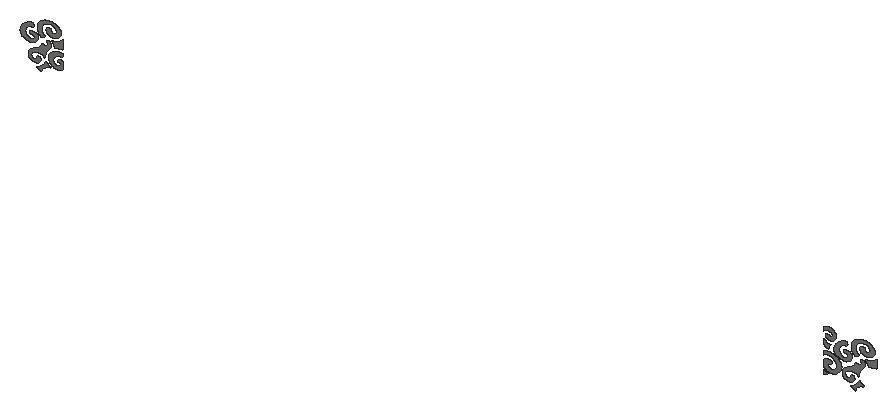
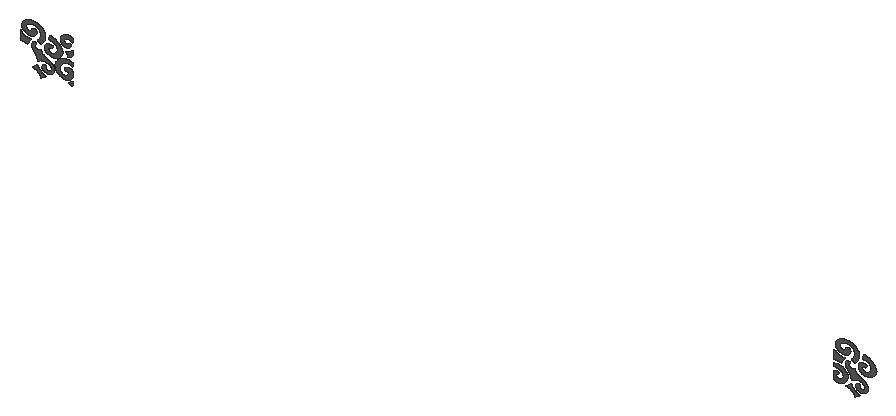
# SketchUp Ruby script. Lengths in inches.
U = 1.inch
M = Sketchup.active_model
def pt(a) = Geom::Point3d.new(a.map { |v| v * U })
def face(e, loops, mat)
  f = e.add_face(loops[0].map { |a| pt(a) })
  loops[1..].each { |l| e.add_face(l.map { |a| pt(a) }).erase! }
  f.material = f.back_material = mat if mat
  f
end
# faces: each face lists its corners as indices into pts; further lists are holes
def faces(e, pts, list, mat = nil) = list.each { |f| face(e, (f[0].is_a?(Array) ? f : [f]).map { |l| l.map { |i| pts[i] } }, mat) }
# xy, xz, yz: faces in a plane at the given z, y or x. An outline is a flat list of corners, or four numbers for a rectangle; further outlines are holes
def ring(l) = l.size == 4 ? [[l[0], l[1]], [l[2], l[1]], [l[2], l[3]], [l[0], l[3]]] : l.each_slice(2).to_a
def flat(e, list, mat, &to3) = list.each { |f| face(e, (f[0].is_a?(Array) ? f : [f]).map { |l| ring(l).map { |u, v| to3.(u, v) } }, mat) }
def xy(e, z, list, mat = nil) = flat(e, list, mat) { |x, y| [x, y, z] }
def xz(e, y, list, mat = nil) = flat(e, list, mat) { |x, z| [x, y, z] }
def yz(e, x, list, mat = nil) = flat(e, list, mat) { |y, z| [x, y, z] }
def lines(e, pts, list) = list.each { |a, b| e.add_line(pt(pts[a]), pt(pts[b])) }
# prism: a flat outline (further loops are holes) pulled along v
def prism(e, loops, v, mat = nil)
  f = face(e, loops, mat); d = Geom::Vector3d.new(v.map { |x| x * U })
  f.pushpull(f.normal.samedirection?(d) ? d.length : -d.length)
end
def box(e, o, s, mat = nil) = prism(e, [[o, [o[0] + s[0], o[1], o[2]], [o[0] + s[0], o[1] + s[1], o[2]], [o[0], o[1] + s[1], o[2]]]], [0, 0, s[2]], mat)
def at(x, y, z, deg = 0) = Geom::Transformation.translation(pt([x, y, z])) * Geom::Transformation.rotation(ORIGIN, Z_AXIS, deg.degrees)
def axes(o, x, y, z) = Geom::Transformation.new([*x, 0, *y, 0, *z, 0, *pt(o).to_a, 1])
def part(name) = M.definitions.add(name)
# library, detail: a bought-in or finely detailed component or shape, given as its bounding box
def library(name, o, s) = part(name).tap { |d| box(d.entities, o, s) }
def detail(e, o, s) = box(e.add_group.entities, o, s)
def put(e, d, t, mat = nil) = e.add_instance(d, t).tap { |i| i.material = mat if mat }
def group(e, t, mat = nil) = e.add_group.tap { |g| g.transformation = t; g.material = mat if mat }.entities
root = M.entities
M.materials.add("[0043_SaddleBrown]4").color = [124, 123, 122]
xz(root,589.17,[[1666.8,173.83,1666.31,174.24,1665.8125,174.64,1665.29,175.02,1664.75,175.39,1664.1875,175.74,1663.61,176.08,1663.01,176.4,1662.4,176.71,1661.77,177,1661.13,177.27,1660.48,177.53,1659.8125,177.77,1661.375,178.34,1662.88,178.99,1664.3125,179.72,1665.67,180.52,1666.95,181.39,1668.14,182.32,1669.23,183.31,1670.22,184.35,1671.11,185.44,1671.89,186.58,1672.55,187.75,1673.1,188.95,1673.65,188.49,1674.21,188.03,1674.78,187.59,1675.36,187.15,1675.95,186.72,1676.55,186.29,1677.17,185.87,1677.79,185.46,1678.41,185.06,1679.05,184.66,1679.7,184.27,1680.36,183.89,1678.69,183.57,1677.08,183.14,1675.54,182.59,1674.08,181.94,1672.71,181.19,1671.46,180.35,1670.32,179.42,1669.32,178.41,1668.46,177.34,1667.74,176.21,1667.19,175.04],[2917.42,173.83,2916.94,174.24,2916.4375,174.64,2915.91,175.02,2915.37,175.39,2914.8125,175.74,2914.23,176.08,2913.64,176.4,2913.03,176.71,2912.4,177,2911.76,177.27,2911.1,177.53,2910.4375,177.77,2912,178.34,2913.5,178.99,2914.9375,179.72,2916.3,180.52,2917.57,181.39,2918.76,182.32,2919.85,183.31,2920.85,184.35,2921.73,185.44,2922.51,186.58,2923.18,187.75,2923.72,188.95,2924.27,188.49,2924.83,188.03,2925.99,187.15,2926.58,186.72,2927.18,186.29,2927.79,185.87,2928.41,185.46,2929.04,185.06,2929.68,184.66,2930.32,184.27,2930.98,183.89,2929.32,183.57,2927.71,183.14,2926.17,182.59,2924.7,181.94,2923.34,181.19,2922.08,180.35,2920.95,179.42,2919.94,178.41,2919.08,177.34,2918.37,176.21,2917.81,175.04],[2869.23,179.89,2869.23,185.26,2869.64,184.92,2870.08,184.6,2870.53,184.3,2871.01,184.01,2871.5,183.73,2872.01,183.47,2872.53,183.23,2873.07,183,2873.62,182.79,2874.18,182.6,2874.76,182.42,2875.34,182.27,2874.96,181.9375,2874.55,181.63,2874.11,181.34,2873.64,181.07,2873.15,180.83,2872.63,180.61,2872.1,180.42,2871.55,180.26,2870.98,180.12,2870.4,180.02,2869.82,179.9375],[1656.02,183.24,1654.59,183.36,1653.2,183.65,1651.89,184.08,1650.68,184.65,1649.61,185.34,1648.69,186.15,1647.96,187.04,1647.42,188.01,1647.09,189.02,1646.98,190.0625,1646.87,191.26,1646.93,192.46,1647.17,193.65,1647.57,194.8125,1648.14,195.9375,1648.86,197.02,1649.74,198.04,1650.76,198.99,1651.91,199.85,1653.18,200.63,1654.56,201.31,1656.02,201.88,1657.41,202.4,1658.74,202.99,1660.02,203.65,1661.22,204.37,1662.35,205.15,1663.4,205.98,1664.37,206.87,1665.25,207.81,1666.03,208.78,1666.71,209.8,1667.3,210.85,1667.77,211.92,1668.45,211.55,1669.19,211.25,1669.98,211.03,1670.81,210.88,1671.65,210.82,1672.5,210.84,1673.34,210.9375,1674.15,211.12,1674.92,211.38,1675.63,211.72,1676.28,212.12,1676.84,212.58,1677.05,212.95,1677.19,213.33,1677.28,213.73,1677.3,214.13,1677.26,214.53,1677.16,214.92,1677,215.3,1676.78,215.67,1676.5,216.02,1676.17,216.34,1675.79,216.63,1675.37,216.89,1675.14,217.04,1674.96,217.23,1674.83,217.43,1674.75,217.65,1674.74,217.875,1674.79,218.1,1674.9,218.3125,1675.07,218.5,1675.28,218.67,1675.53,218.8,1675.82,218.9,1676.12,218.95,1676.68,218.98,1677.23,218.95,1677.78,218.86,1678.3,218.72,1678.79,218.52,1679.23,218.28,1679.625,217.99,1679.96,217.67,1680.22,217.3125,1680.41,216.9375,1680.53,216.54,1680.57,216.14,1680.78,215.47,1680.93,214.79,1681,214.11,1681.01,213.42,1680.95,212.73,1680.82,212.05,1680.62,211.38,1680.35,210.72,1680.02,210.08,1679.62,209.45,1679.16,208.85,1678.64,208.27,1677.71,207.26,1676.84,206.23,1676.03,205.16,1675.29,204.07,1674.63,202.95,1674.03,201.82,1673.51,200.67,1673.05,199.5,1672.68,198.32,1672.375,197.12,1672.15,195.92,1672,194.71,1671.03,195.61,1669.91,196.41,1668.65,197.09,1667.29,197.66,1665.83,198.09,1664.31,198.375,1662.74,198.52,1661.17,198.52,1659.61,198.37,1658.09,198.07,1656.63,197.63,1655.27,197.0625,1654.29,196.53,1653.43,195.9,1652.68,195.2,1652.06,194.44,1651.58,193.625,1651.25,192.77,1651.07,191.9,1651.06,191.01,1651.2,190.14,1651.5,189.28,1651.94,188.46,1652.53,187.68,1653.08,187.38,1653.68,187.15,1654.32,186.98,1654.99,186.89,1655.68,186.87,1656.36,186.92,1657.02,187.04,1657.64,187.24,1658.23,187.5,1658.75,187.82,1659.19,188.1875,1659.5625,188.6,1659.44,188.9,1659.35,189.2,1659.3,189.5,1659.28,189.81,1659.3,190.12,1659.34,190.42,1659.42,190.72,1659.54,191.02,1659.69,191.31,1659.86,191.59,1660.07,191.86,1660.31,192.11,1660.54,192.31,1660.8125,192.48,1661.12,192.61,1661.45,192.71,1661.8,192.77,1662.15,192.79,1662.51,192.77,1662.86,192.71,1663.19,192.61,1663.5,192.48,1663.77,192.31,1664,192.11,1664.67,191.31,1665.15,190.43,1665.4,189.51,1665.4375,188.57,1665.25,187.63,1664.84,186.74,1664.23,185.91,1663.43,185.17,1662.46,184.53,1661.36,184.03,1660.16,183.66,1658.89,183.45,1657.47,183.27],[2906.65,183.24,2905.21,183.36,2903.83,183.65,2902.51,184.08,2901.3,184.65,2900.23,185.34,2899.32,186.15,2898.58,187.04,2898.04,188.01,2897.72,189.02,2897.61,190.0625,2897.49,191.26,2897.56,192.46,2897.79,193.65,2898.19,194.8125,2898.76,195.9375,2899.49,197.02,2900.37,198.04,2901.39,198.99,2902.54,199.85,2903.81,200.63,2905.18,201.31,2906.65,201.88,2908.04,202.4,2909.37,202.99,2910.64,203.65,2911.85,204.37,2912.98,205.15,2914.03,205.98,2914.99,206.87,2915.87,207.81,2916.65,208.78,2917.34,209.8,2917.92,210.85,2918.4,211.92,2919.08,211.55,2919.82,211.25,2920.61,211.03,2921.43,210.88,2922.28,210.82,2923.13,210.84,2923.97,210.9375,2924.78,211.12,2925.55,211.38,2926.26,211.72,2926.9,212.12,2927.47,212.58,2927.67,212.95,2927.82,213.33,2927.9,213.73,2927.93,214.13,2927.89,214.53,2927.78,214.92,2927.62,215.3,2927.4,215.67,2927.125,216.02,2926.79,216.34,2926.42,216.63,2926,216.89,2925.77,217.04,2925.58,217.23,2925.45,217.43,2925.38,217.65,2925.37,217.875,2925.42,218.1,2925.53,218.3125,2925.69,218.5,2925.9,218.67,2926.16,218.8,2926.44,218.9,2926.75,218.95,2927.3,218.98,2927.86,218.95,2928.4,218.86,2928.93,218.72,2929.41,218.52,2929.86,218.28,2930.25,217.99,2930.58,217.67,2930.85,217.3125,2931.04,216.9375,2931.16,216.54,2931.19,216.14,2931.41,215.47,2931.55,214.79,2931.63,214.11,2931.64,213.42,2931.57,212.73,2931.44,212.05,2931.24,211.38,2930.98,210.72,2930.64,210.08,2930.24,209.45,2929.79,208.85,2929.27,208.27,2928.33,207.26,2927.46,206.23,2926.66,205.16,2925.92,204.07,2925.25,202.95,2924.66,201.82,2924.13,200.67,2923.68,199.5,2923.3,198.32,2923,197.12,2922.77,195.92,2922.62,194.71,2921.65,195.61,2920.53,196.41,2919.28,197.09,2917.91,197.66,2916.45,198.09,2914.93,198.375,2913.37,198.52,2911.79,198.52,2910.23,198.37,2908.71,198.07,2907.26,197.63,2905.89,197.0625,2904.92,196.53,2904.05,195.9,2903.3,195.2,2902.68,194.44,2902.2,193.625,2901.875,192.77,2901.7,191.9,2901.68,191.01,2901.82,190.14,2902.12,189.28,2902.57,188.46,2903.16,187.68,2903.7,187.38,2904.31,187.15,2904.95,186.98,2905.62,186.89,2906.3,186.87,2906.98,186.92,2907.64,187.04,2908.27,187.24,2908.85,187.5,2909.37,187.82,2909.82,188.1875,2910.1875,188.6,2910.07,188.9,2909.98,189.2,2909.93,189.5,2909.91,189.81,2909.92,190.12,2909.97,190.42,2910.05,190.72,2910.16,191.02,2910.31,191.31,2910.49,191.59,2910.7,191.86,2910.93,192.11,2911.16,192.31,2911.4375,192.48,2911.74,192.61,2912.07,192.71,2912.42,192.77,2912.78,192.79,2913.14,192.77,2913.48,192.71,2913.82,192.61,2914.12,192.48,2914.39,192.31,2914.625,192.11,2915.3,191.31,2915.77,190.43,2916.03,189.51,2916.0625,188.57,2915.875,187.63,2915.47,186.74,2914.85,185.91,2914.05,185.17,2913.09,184.53,2911.99,184.03,2910.78,183.66,2909.51,183.45,2908.09,183.27],
  [2879.38,184.38,2878.22,184.54,2877.08,184.78,2875.99,185.09,2874.9375,185.48,2873.94,185.94,2873.01,186.47,2872.16,187.05,2871.38,187.69,2870.7,188.38,2870.11,189.12,2869.61,189.89,2869.23,190.7,2869.23,198.78,2869.76,199.6875,2870.53,200.5,2871.52,201.17,2872.68,201.69,2873.96,202.03,2875.3,202.17,2876.67,202.12,2877.98,201.86,2879.2,201.42,2880.26,200.8,2881.13,200.05,2881.77,199.18,2881.87,198.97,2881.92,198.75,2881.92,198.53,2881.88,198.32,2881.8,198.1,2881.67,197.9,2881.51,197.72,2881.31,197.55,2881.07,197.41,2880.82,197.3,2880.54,197.21,2880.24,197.15,2879.51,197.24,2878.78,197.23,2878.06,197.13,2877.375,196.93,2876.75,196.64,2876.22,196.28,2875.78,195.85,2875.47,195.37,2875.28,194.85,2875.22,194.32,2875.31,193.8,2875.52,193.29,2875.7,192.63,2876.03,192,2876.49,191.41,2877.07,190.88,2877.76,190.43,2878.53,190.06,2879.38,189.78,2880.28,189.6,2881.21,189.53,2882.14,189.5625,2883.06,189.7,2883.93,189.9375,2885.28,190.72,2886.47,191.64,2887.47,192.67,2888.25,193.79,2888.8125,194.98,2889.13,196.21,2889.2,197.47,2889.03,198.72,2888.61,199.93,2887.96,201.1,2887.09,202.18,2886.01,203.17,2885.57,203.82,2885.06,204.45,2884.47,205.04,2883.83,205.59,2883.12,206.1,2882.35,206.57,2881.53,206.99,2880.67,207.37,2879.76,207.68,2878.82,207.94,2877.86,208.15,2876.875,208.3,2876.17,208.36,2875.47,208.375,2874.76,208.35,2874.0625,208.28,2873.37,208.17,2872.7,208.02,2872.04,207.83,2871.41,207.6,2870.8125,207.33,2870.24,207.03,2869.71,206.69,2869.23,206.32,2869.23,211.9,2871.37,212.41,2873.59,212.74,2875.84,212.875,2878.1,212.8125,2880.34,212.56,2882.51,212.11,2884.6,211.48,2886.5625,210.67,2888.38,209.7,2890.02,208.58,2891.47,207.33,2892.7,205.96,2894.37,203.92,2895.52,201.7,2896.14,199.375,2896.18,197.01,2895.66,194.67,2894.59,192.43,2893,190.36,2890.9375,188.51,2888.46,186.95,2885.66,185.72,2882.6,184.86],[1691.55,185,1690.19,185.0625,1688.86,185.24,1687.5625,185.54,1686.33,185.94,1685.17,186.46,1684.11,187.07,1683.22,187.69,1682.38,188.36,1681.61,189.0625,1680.91,189.8,1680.28,190.57,1679.72,191.375,1679.23,192.2,1678.83,193.05,1678.5,193.92,1678.26,194.79,1678.09,195.68,1678.01,196.58,1678.13,198.46,1678.64,200.32,1679.53,202.09,1680.78,203.75,1682.36,205.26,1684.24,206.58,1686.37,207.67,1688.7,208.53,1691.19,209.12,1693.78,209.4375,1696.39,209.47,1698.99,209.22,1698.99,204.51,1696.76,204.57,1694.55,204.34,1692.43,203.84,1690.46,203.08,1688.71,202.09,1687.22,200.89,1686.04,199.53,1685.21,198.03,1684.75,196.46,1684.67,194.85,1684.99,193.26,1685.6875,191.73,1686.48,191.08,1687.43,190.54,1688.51,190.15,1689.67,189.91,1690.87,189.83,1692.07,189.91,1693.23,190.16,1694.3,190.55,1695.25,191.09,1696.04,191.75,1696.65,192.5,1697.05,193.32,1697.125,193.65,1697.12,193.99,1697.03,194.32,1696.87,194.64,1696.63,194.93,1696.33,195.19,1695.97,195.4,1695.5625,195.57,1695.125,195.6875,1694.66,195.75,1694.2,195.75,1693.73,195.7,1693.49,195.77,1693.26,195.87,1693.05,195.98,1692.86,196.11,1692.68,196.25,1692.53,196.41,1692.4,196.58,1692.3,196.75,1692.22,196.93,1692.17,197.12,1692.15,197.3125,1692.16,197.5,1692.53,197.89,1692.97,198.24,1693.46,198.54,1694.01,198.8,1694.6,199,1695.23,199.14,1695.87,199.22,1696.52,199.24,1697.17,199.19,1697.8,199.09,1698.42,198.93,1698.99,198.7,1698.99,187.07,1697.93,186.46,1696.77,185.94,1695.54,185.54,1694.24,185.24,1692.91,185.0625],[1649.44,208.61,1647.11,208.71,1644.82,209.07,1642.64,209.68,1640.62,210.53,1638.8125,211.6,1637.25,212.86,1635.99,214.28,1635.04,215.82,1634.44,217.45,1634.2,219.125,1634.33,220.81,1634.82,222.46,1635.375,224.06,1636.13,225.62,1637.08,227.12,1638.22,228.55,1639.54,229.9,1641.02,231.16,1642.66,232.31,1644.44,233.35,1646.34,234.27,1648.35,235.06,1650.45,235.71,1652.625,236.22,1653.04,235.77,1653.4,235.31,1653.71,234.82,1653.98,234.32,1654.1875,233.81,1654.34,233.28,1654.44,232.75,1654.49,232.22,1654.48,231.68,1654.41,231.15,1654.29,230.62,1654.12,230.1,1652.76,230.21,1651.4,230.19,1650.06,230.04,1648.76,229.75,1647.53,229.33,1646.38,228.8,1645.36,228.16,1644.46,227.42,1643.71,226.6,1643.13,225.71,1642.72,224.77,1642.5,223.8,1642.13,222.89,1641.9,221.95,1641.8125,221,1641.87,220.05,1642.06,219.11,1642.39,218.19,1642.86,217.3,1643.45,216.45,1644.17,215.65,1645.01,214.91,1645.94,214.24,1646.98,213.65,1647.93,213.25,1648.98,212.99,1650.07,212.875,1651.18,212.91,1652.25,213.1,1653.26,213.43,1654.16,213.89,1654.93,214.46,1655.53,215.13,1655.94,215.875,1656.16,216.66,1656.16,217.45,1656.07,217.85,1655.91,218.23,1655.68,218.59,1655.38,218.92,1655.03,219.23,1654.61,219.49,1654.16,219.71,1653.66,219.89,1653.14,220.01,1652.6,220.09,1652.04,220.1,1651.49,220.07,1650.92,220.05,1650.36,220.13,1649.83,220.3,1649.37,220.55,1649,220.86,1648.75,221.23,1648.61,221.63,1648.61,222.05,1648.73,222.45,1648.98,222.83,1649.34,223.15,1649.79,223.4,1651.04,223.84,1652.38,224.12,1653.76,224.21,1655.14,224.12,1656.48,223.85,1657.73,223.4,1658.84,222.81,1659.79,222.07,1660.53,221.23,1661.06,220.3,1661.33,219.32,1661.36,218.32,1661.41,217.11,1661.24,215.9,1660.83,214.72,1660.21,213.6,1659.375,212.54,1658.35,211.58,1657.15,210.73,1655.8,210.01,1654.33,209.42,1652.76,208.99,1651.12,208.72],[2900.07,208.61,2897.73,208.71,2895.45,209.07,2893.27,209.68,2891.25,210.53,2889.4375,211.6,2887.88,212.86,2886.61,214.28,2885.67,215.82,2885.07,217.45,2884.83,219.125,2884.96,220.81,2885.45,222.46,2886,224.06,2886.76,225.62,2887.71,227.12,2888.85,228.55,2890.16,229.9,2891.65,231.16,2893.28,232.31,2895.06,233.35,2896.96,234.27,2898.97,235.06,2901.07,235.71,2903.25,236.22,2903.66,235.77,2904.03,235.31,2904.34,234.82,2904.6,234.32,2904.8125,233.81,2904.97,233.28,2905.07,232.75,2905.11,232.22,2905.1,231.68,2905.04,231.15,2904.92,230.62,2904.74,230.1,2903.39,230.21,2902.03,230.19,2900.69,230.04,2899.38,229.75,2898.15,229.33,2897.01,228.8,2895.98,228.16,2895.08,227.42,2894.34,226.6,2893.76,225.71,2893.35,224.77,2893.125,223.8,2892.76,222.89,2892.53,221.95,2892.4375,221,2892.49,220.05,2892.68,219.11,2893.02,218.19,2893.48,217.3,2894.08,216.45,2894.8,215.65,2895.63,214.91,2896.57,214.24,2897.6,213.65,2898.56,213.25,2899.6,212.99,2900.7,212.875,2901.8,212.91,2902.875,213.1,2903.88,213.43,2904.79,213.89,2905.55,214.46,2906.15,215.13,2906.57,215.875,2906.78,216.66,2906.78,217.45,2906.7,217.85,2906.54,218.23,2906.31,218.59,2906.01,218.92,2905.65,219.23,2905.24,219.49,2904.78,219.71,2904.29,219.89,2903.76,220.01,2903.22,220.09,2902.67,220.1,2902.12,220.07,2901.55,220.05,2900.98,220.13,2900.46,220.3,2900,220.55,2899.63,220.86,2899.37,221.23,2899.24,221.63,2899.23,222.05,2899.36,222.45,2899.61,222.83,2899.97,223.15,2900.42,223.4,2901.66,223.84,2903,224.12,2904.39,224.21,2905.77,224.12,2907.11,223.85,2908.35,223.4,2909.47,222.81,2910.41,222.07,2911.16,221.23,2911.68,220.3,2911.96,219.32,2911.98,218.32,2912.04,217.11,2911.86,215.9,2911.46,214.72,2910.83,213.6,2910,212.54,2908.98,211.58,2907.78,210.73,2906.43,210.01,2904.95,209.42,2903.38,208.99,2901.74,208.72],[1687.01,213.07,1686.91,213.85,1686.75,214.62,1686.53,215.39,1686.27,216.14,1685.95,216.89,1685.57,217.625,1685.15,218.34,1684.68,219.05,1684.15,219.73,1683.58,220.4,1682.97,221.04,1682.31,221.66,1683.96,221.55,1685.62,221.5625,1687.27,221.7,1688.89,221.96,1690.47,222.33,1691.99,222.82,1693.43,223.41,1694.78,224.11,1696.02,224.91,1697.14,225.79,1698.14,226.75,1698.99,227.78,1698.99,215.23,1697.95,215.21,1696.92,215.16,1695.88,215.08,1694.85,214.98,1693.83,214.84,1692.82,214.67,1691.82,214.47,1690.83,214.25,1689.85,213.99,1688.89,213.71,1687.9375,213.41],
  [2937.63,213.07,2937.53,213.85,2937.37,214.62,2937.16,215.39,2936.89,216.14,2936.57,216.89,2936.2,217.625,2935.78,218.34,2935.3,219.05,2934.78,219.73,2934.21,220.4,2933.59,221.04,2932.93,221.66,2934.59,221.55,2936.25,221.5625,2937.9,221.7,2939.52,221.96,2941.1,222.33,2942.61,222.82,2944.05,223.41,2945.4,224.11,2946.64,224.91,2947.77,225.79,2948.76,226.75,2949.62,227.78,2949.62,215.23,2948.58,215.21,2947.54,215.16,2946.51,215.08,2945.48,214.98,2944.46,214.84,2943.45,214.67,2942.44,214.47,2941.45,214.25,2940.47,213.99,2939.51,213.71,2938.5625,213.41],[2876.57,216.375,2875.87,216.63,2875.19,216.91,2874.51,217.2,2873.86,217.52,2873.22,217.84,2872.59,218.1875,2871.98,218.54,2871.39,218.92,2870.82,219.31,2870.27,219.71,2869.74,220.125,2869.23,220.56,2869.23,227.67,2869.75,227.04,2870.34,226.43,2870.99,225.86,2871.71,225.34,2872.49,224.85,2873.32,224.42,2874.19,224.03,2875.11,223.7,2876.06,223.42,2877.03,223.2,2878.03,223.04,2879.05,222.93,2878.63,222.44,2878.25,221.9375,2877.9,221.42,2877.6,220.89,2877.33,220.35,2877.1,219.79,2876.91,219.23,2876.76,218.67,2876.65,218.1,2876.58,217.52,2876.55,216.95],[1666.39,220.74,1665.27,221.82,1664.26,222.95,1663.37,224.13,1662.6,225.36,1661.97,226.63,1661.46,227.92,1661.1,229.24,1660.86,230.58,1660.77,231.92,1660.82,233.27,1661,234.61,1661.32,235.94,1661.85,237.37,1662.58,238.75,1663.5,240.07,1664.61,241.32,1665.88,242.48,1667.32,243.55,1668.89,244.5,1670.59,245.33,1672.4,246.03,1674.3,246.59,1676.27,247.02,1678.29,247.29,1680.49,247.4,1682.69,247.29,1684.85,246.97,1686.93,246.4375,1688.89,245.71,1690.7,244.79,1692.31,243.71,1693.71,242.47,1694.86,241.12,1695.74,239.66,1696.34,238.125,1696.64,236.55,1696.64,235.18,1696.36,233.83,1695.8,232.52,1694.99,231.29,1693.93,230.15,1692.66,229.14,1691.19,228.27,1689.57,227.57,1687.82,227.04,1685.98,226.71,1684.09,226.57,1682.2,226.63,1680.72,226.85,1679.32,227.24,1678.02,227.79,1676.87,228.48,1675.89,229.3,1675.11,230.23,1674.54,231.23,1674.22,232.29,1674.14,233.37,1674.3,234.45,1674.71,235.49,1675.35,236.47,1675.87,236.87,1676.48,237.18,1677.17,237.39,1677.91,237.5,1678.66,237.49,1679.4,237.375,1680.09,237.15,1680.69,236.83,1681.2,236.43,1681.57,235.96,1681.81,235.44,1681.7,235.09,1681.64,234.73,1681.63,234.37,1681.6875,234.01,1681.8,233.65,1681.96,233.3125,1682.18,232.98,1682.44,232.68,1682.75,232.39,1683.11,232.13,1683.5,231.91,1683.92,231.71,1684.93,231.82,1685.91,232.03,1686.83,232.35,1687.67,232.77,1688.41,233.28,1689.04,233.86,1689.53,234.5,1689.88,235.19,1690.08,235.91,1690.125,236.65,1690.01,237.38,1689.74,238.09,1689,239.28,1687.99,240.36,1686.74,241.3,1685.29,242.08,1683.6875,242.67,1681.97,243.07,1680.18,243.25,1678.37,243.21,1676.6,242.96,1674.91,242.5,1673.35,241.84,1671.97,241,1670.52,239.82,1669.3,238.51,1668.32,237.1,1667.62,235.6,1667.1875,234.06,1667.04,232.48,1667.1875,230.91,1667.62,229.36,1668.32,227.86,1669.3,226.45,1670.52,225.14,1671.97,223.96,1671.61,223.61,1671.22,223.28,1670.82,222.95,1670.39,222.65,1669.95,222.35,1669.49,222.07,1669.01,221.81,1668.51,221.5625,1668,221.33,1667.48,221.12,1666.94,220.92],[2917.02,220.74,2915.89,221.82,2914.88,222.95,2913.99,224.13,2913.23,225.36,2912.59,226.63,2912.09,227.92,2911.72,229.24,2911.49,230.58,2911.4,231.92,2911.44,233.27,2911.625,234.61,2911.95,235.94,2912.48,237.37,2913.21,238.75,2914.13,240.07,2915.23,241.32,2916.51,242.48,2917.94,243.55,2919.51,244.5,2921.22,245.33,2923.02,246.03,2924.92,246.59,2926.89,247.02,2928.91,247.29,2931.11,247.4,2933.31,247.29,2935.48,246.97,2937.56,246.4375,2939.52,245.71,2941.32,244.79,2942.94,243.71,2944.33,242.47,2945.48,241.12,2946.36,239.66,2946.96,238.125,2947.27,236.55,2947.26,235.18,2946.98,233.83,2946.43,232.52,2945.61,231.29,2944.56,230.15,2943.29,229.14,2941.82,228.27,2940.19,227.57,2938.44,227.04,2936.6,226.71,2934.72,226.57,2932.82,226.63,2931.35,226.85,2929.94,227.24,2928.65,227.79,2927.49,228.48,2926.51,229.3,2925.73,230.23,2925.17,231.23,2924.84,232.29,2924.76,233.37,2924.93,234.45,2925.34,235.49,2925.98,236.47,2926.49,236.87,2927.11,237.18,2927.8,237.39,2928.54,237.5,2929.29,237.49,2930.02,237.375,2930.71,237.15,2931.32,236.83,2931.82,236.43,2932.2,235.96,2932.43,235.44,2932.32,235.09,2932.26,234.73,2932.26,234.37,2932.3125,234.01,2932.42,233.65,2932.59,233.3125,2932.8,232.98,2933.07,232.68,2933.38,232.39,2933.73,232.13,2934.125,231.91,2934.55,231.71,2935.56,231.82,2936.54,232.03,2937.46,232.35,2938.3,232.77,2939.04,233.28,2939.66,233.86,2940.16,234.5,2940.51,235.19,2940.71,235.91,2940.75,236.65,2940.64,237.38,2940.37,238.09,2939.62,239.28,2938.61,240.36,2937.36,241.3,2935.92,242.08,2934.3125,242.67,2932.59,243.07,2930.8,243.25,2929,243.21,2927.23,242.96,2925.54,242.5,2923.98,241.84,2922.6,241,2921.15,239.82,2919.92,238.51,2918.95,237.1,2918.24,235.6,2917.8125,234.06,2917.67,232.48,2917.8125,230.91,2918.24,229.36,2918.95,227.86,2919.92,226.45,2921.15,225.14,2922.6,223.96,2922.23,223.61,2921.85,223.28,2921.44,222.95,2921.02,222.65,2920.58,222.35,2920.11,222.07,2919.63,221.81,2919.14,221.5625,2918.63,221.33,2918.1,221.12,2917.57,220.92],[2879.08,229.18,2877.8,229.23,2876.55,229.45,2875.38,229.84,2874.34,230.38,2873.46,231.06,2872.77,231.84,2872.29,232.7,2872.05,233.61,2871.96,233.96,2871.97,234.32,2872.07,234.67,2872.26,235,2872.54,235.29,2872.9,235.54,2873.31,235.74,2873.77,235.875,2874.25,235.94,2874.75,235.94,2875.24,235.87,2875.69,235.73,2875.96,235.48,2876.25,235.24,2876.56,235.01,2876.89,234.8,2877.23,234.6,2877.6,234.42,2877.97,234.26,2878.37,234.11,2878.77,233.98,2879.18,233.87,2879.61,233.78,2880.03,233.71,2880.6,234.05,2881.1,234.45,2881.53,234.89,2881.875,235.36,2882.15,235.86,2882.33,236.375,2882.42,236.91,2882.42,237.44,2882.33,237.97,2882.15,238.49,2881.89,238.99,2881.54,239.46,2880.8125,240.18,2879.93,240.79,2878.91,241.29,2877.79,241.65,2876.61,241.875,2875.38,241.95,2874.16,241.875,2872.97,241.65,2871.85,241.29,2870.84,240.79,2869.95,240.18,2869.23,239.46,2869.23,244.71,2870.1,245.16,2871.03,245.55,2872.01,245.87,2873.03,246.125,2874.08,246.3,2875.15,246.41,2876.22,246.4375,2877.3,246.39,2878.36,246.27,2879.4,246.08,2880.42,245.8125,2881.39,245.48,2883.08,244.68,2884.58,243.71,2885.84,242.57,2886.83,241.3,2887.53,239.93,2887.91,238.5,2887.97,237.04,2887.71,235.6,2887.13,234.2,2886.24,232.89,2885.08,231.7,2883.67,230.65,2882.6875,230.05,2881.57,229.6,2880.35,229.3]],"[0043_SaddleBrown]4")
p = [[2932.52,589.17,234.9],[2932.43,589.17,235.44],[2869.23,589.17,176.23],[2869.23,589.17,179.89],[1681.89,589.17,234.9],[1681.81,589.17,235.44]]
lines(root,p,[[0,1],[2,3],[4,5]])
